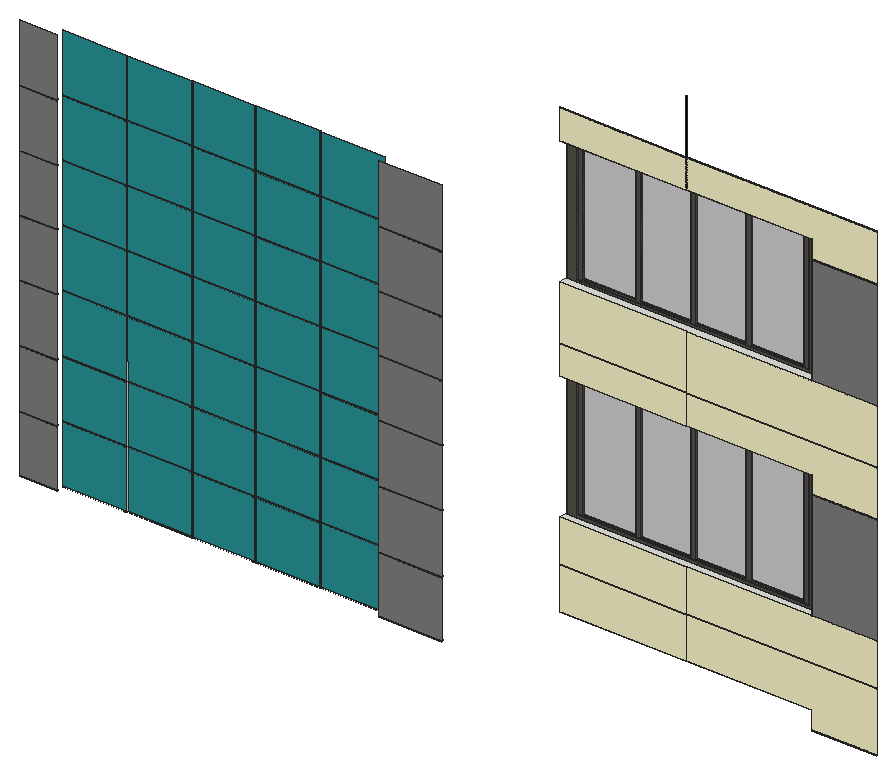
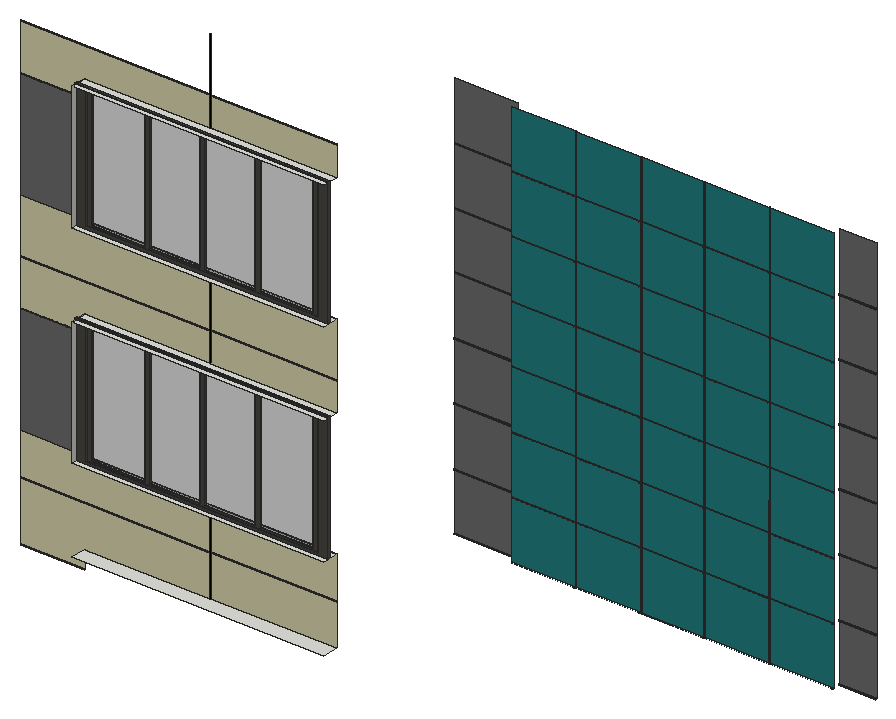
# SketchUp Ruby script. Lengths in inches.
U = 1.inch
M = Sketchup.active_model
def pt(a) = Geom::Point3d.new(a.map { |v| v * U })
def face(e, loops, mat)
  f = e.add_face(loops[0].map { |a| pt(a) })
  loops[1..].each { |l| e.add_face(l.map { |a| pt(a) }).erase! }
  f.material = f.back_material = mat if mat
  f
end
# faces: each face lists its corners as indices into pts; further lists are holes
def faces(e, pts, list, mat = nil) = list.each { |f| face(e, (f[0].is_a?(Array) ? f : [f]).map { |l| l.map { |i| pts[i] } }, mat) }
# xy, xz, yz: faces in a plane at the given z, y or x. An outline is a flat list of corners, or four numbers for a rectangle; further outlines are holes
def ring(l) = l.size == 4 ? [[l[0], l[1]], [l[2], l[1]], [l[2], l[3]], [l[0], l[3]]] : l.each_slice(2).to_a
def flat(e, list, mat, &to3) = list.each { |f| face(e, (f[0].is_a?(Array) ? f : [f]).map { |l| ring(l).map { |u, v| to3.(u, v) } }, mat) }
def xy(e, z, list, mat = nil) = flat(e, list, mat) { |x, y| [x, y, z] }
def xz(e, y, list, mat = nil) = flat(e, list, mat) { |x, z| [x, y, z] }
def yz(e, x, list, mat = nil) = flat(e, list, mat) { |y, z| [x, y, z] }
def lines(e, pts, list) = list.each { |a, b| e.add_line(pt(pts[a]), pt(pts[b])) }
# prism: a flat outline (further loops are holes) pulled along v
def prism(e, loops, v, mat = nil)
  f = face(e, loops, mat); d = Geom::Vector3d.new(v.map { |x| x * U })
  f.pushpull(f.normal.samedirection?(d) ? d.length : -d.length)
end
def box(e, o, s, mat = nil) = prism(e, [[o, [o[0] + s[0], o[1], o[2]], [o[0] + s[0], o[1] + s[1], o[2]], [o[0], o[1] + s[1], o[2]]]], [0, 0, s[2]], mat)
def at(x, y, z, deg = 0) = Geom::Transformation.translation(pt([x, y, z])) * Geom::Transformation.rotation(ORIGIN, Z_AXIS, deg.degrees)
def axes(o, x, y, z) = Geom::Transformation.new([*x, 0, *y, 0, *z, 0, *pt(o).to_a, 1])
def part(name) = M.definitions.add(name)
# library, detail: a bought-in or finely detailed component or shape, given as its bounding box
def library(name, o, s) = part(name).tap { |d| box(d.entities, o, s) }
def detail(e, o, s) = box(e.add_group.entities, o, s)
def put(e, d, t, mat = nil) = e.add_instance(d, t).tap { |i| i.material = mat if mat }
def group(e, t, mat = nil) = e.add_group.tap { |g| g.transformation = t; g.material = mat if mat }.entities
root = M.entities
M.materials.add("Aluminum_Anodized_DarkGray").color = [87, 83, 78]
M.materials.add("Glass_Coated_Black").color = [65, 65, 65]
M.materials["Glass_Coated_Black"].alpha = 0.42
M.materials.add("[0050_LemonChiffon]").color = [255, 250, 205]
M.materials.add("[0081_CadetBlue]").color = [40, 149, 153]
M.materials.add("[0133_Gray]").color = [128, 128, 128]
M.materials.add("[0137_Black]").color = [0, 0, 0]
c1 = part("Group\#2")
xy(c1.entities,0,[[0,0,54,3]],"Aluminum_Anodized_DarkGray")
xy(c1.entities,2,[[2.25,0,51.75,1],[2.25,2,51.75,3]],"Aluminum_Anodized_DarkGray")
xy(c1.entities,3,[[3.375,1,14.625,1.5],[15.75,1,26.4375,1.5],[27.5625,1,38.25,1.5],[39.375,1,50.625,1.5],[3.375,1.5,14.625,2],
  [15.75,1.5,26.4375,2],[27.5625,1.5,38.25,2],[39.375,1.5,50.625,2]],"Aluminum_Anodized_DarkGray")
xy(c1.entities,99,[[3.375,1,14.625,1.5],[15.75,1,26.4375,1.5],[26.4375,1,27.5625,2],[27.5625,1,38.25,1.5],[38.25,1,39.375,2],
  [39.375,1,50.625,1.5],[3.375,1.5,14.625,2],[15.75,1.5,26.4375,2],[27.5625,1.5,38.25,2],[39.375,1.5,50.625,2]],"Aluminum_Anodized_DarkGray")
xy(c1.entities,100,[[2.25,0,51.75,1],[2.25,2,51.75,3]],"Aluminum_Anodized_DarkGray")
xy(c1.entities,102,[[0,0,54,3]],"Aluminum_Anodized_DarkGray")
xz(c1.entities,0,[[[0,0,54,102],[2.25,2,51.75,100]]],"Aluminum_Anodized_DarkGray")
xz(c1.entities,1,[[[2.25,2,51.75,100],[39.375,3,50.625,99],[3.375,3,14.625,99],[27.5625,3,38.25,99],[15.75,3,26.4375,99]]],"Aluminum_Anodized_DarkGray")
xz(c1.entities,1.5,[[3.375,3,14.625,99],[15.75,3,27,99],[27.5625,3,38.8125,99],[39.375,3,50.625,99]],"Glass_Coated_Black")
xz(c1.entities,2,[[[2.25,2,51.75,100],[39.375,3,50.625,99],[3.375,3,14.625,99],[27.5625,3,38.25,99],[15.75,3,26.4375,99]]],"Aluminum_Anodized_DarkGray")
xz(c1.entities,3,[[[0,0,54,102],[2.25,2,51.75,100]]],"Aluminum_Anodized_DarkGray")
yz(c1.entities,0,[[0,0,3,102]],"Aluminum_Anodized_DarkGray")
yz(c1.entities,2.25,[[0,2,1,100],[2,2,3,100]],"Aluminum_Anodized_DarkGray")
yz(c1.entities,3.375,[[1,3,1.5,99],[1.5,3,2,99]],"Aluminum_Anodized_DarkGray")
yz(c1.entities,14.625,[[1,3,1.5,99],[1.5,3,2,99]],"Aluminum_Anodized_DarkGray")
yz(c1.entities,15.75,[[1,3,1.5,99],[1.5,3,2,99]],"Aluminum_Anodized_DarkGray")
yz(c1.entities,26.4375,[[1,3,2,99]],"Aluminum_Anodized_DarkGray")
yz(c1.entities,27.5625,[[1,3,1.5,99],[1.5,3,2,99]],"Aluminum_Anodized_DarkGray")
yz(c1.entities,38.25,[[1,3,2,99]],"Aluminum_Anodized_DarkGray")
yz(c1.entities,39.375,[[1,3,1.5,99],[1.5,3,2,99]],"Aluminum_Anodized_DarkGray")
yz(c1.entities,50.625,[[1,3,1.5,99],[1.5,3,2,99]],"Aluminum_Anodized_DarkGray")
yz(c1.entities,51.75,[[0,2,1,100],[2,2,3,100]],"Aluminum_Anodized_DarkGray")
yz(c1.entities,54,[[0,0,3,102]],"Aluminum_Anodized_DarkGray")
p = [[15.75,2,99],[14.625,2,99]]
lines(c1.entities,p,[[0,1]])
xy(root,276.01,[[355.9375,305.1875,499.37,314.1875]])
xy(root,297.46,[[115.9375,221.1875,136.9375,221.6875],[319.9375,221.1875,355.9375,221.6875],[136.79,225.49,173.04,225.6875],[173.33,225.49,210.01,225.6875],[210.51,225.49,246.05,225.6875],
  [246.55,225.49,283.09,225.6875],[283.59,225.49,319.625,225.6875]])
xy(root,297.96,[[115.9375,221.1875,136.9375,221.6875],[319.9375,221.1875,355.9375,221.6875],[136.79,225.49,173.04,225.6875],[173.33,225.49,210.01,225.6875],[210.51,225.49,246.05,225.6875],
  [246.55,225.49,283.09,225.6875],[283.59,225.49,319.625,225.6875]])
xy(root,324,[[355.9375,305.1875,499.37,314.1875]])
xy(root,330.2,[[115.9375,221.1875,136.9375,221.6875],[319.9375,221.1875,355.9375,221.6875]])
xy(root,330.7,[[115.9375,221.1875,136.9375,221.6875],[319.9375,221.1875,355.9375,221.6875],[136.75,225.49,173.04,225.6875],[173.29,225.49,210.01,225.6875],[210.51,225.49,246.05,225.6875],
  [246.55,225.49,283.09,225.6875],[283.59,225.49,319.625,225.6875]])
xy(root,331.2,[[136.75,225.49,173.04,225.6875],[173.29,225.49,210.01,225.6875],[210.51,225.49,246.05,225.6875],[246.55,225.49,283.09,225.6875],[283.59,225.49,319.625,225.6875]])
xy(root,363.94,[[115.9375,221.1875,136.9375,221.6875],[319.9375,221.1875,355.9375,221.6875],[136.71,225.49,173.04,225.6875],[173.25,225.49,210.01,225.6875],[210.51,225.49,246.05,225.6875],
  [246.55,225.49,283.09,225.6875],[283.59,225.49,319.625,225.6875]])
xy(root,364.44,[[115.9375,221.1875,136.9375,221.6875],[319.9375,221.1875,355.9375,221.6875],[136.71,225.49,173.04,225.6875],[173.25,225.49,210.01,225.6875],[210.51,225.49,246.05,225.6875],
  [246.55,225.49,283.09,225.6875],[283.59,225.49,319.625,225.6875]])
xy(root,396,[[355.9375,305.1875,499.37,314.1875]])
xy(root,397.18,[[115.9375,221.1875,136.9375,221.6875],[319.9375,221.1875,355.9375,221.6875],[136.68,225.49,173.04,225.6875],[173.21,225.49,210.01,225.6875],[210.51,225.49,246.05,225.6875],
  [246.55,225.49,283.09,225.6875],[283.59,225.49,319.625,225.6875]])
xy(root,397.68,[[115.9375,221.1875,136.9375,221.6875],[319.9375,221.1875,355.9375,221.6875],[136.67,225.49,173.04,225.6875],[173.21,225.49,210.01,225.6875],[210.51,225.49,246.05,225.6875],
  [246.55,225.49,283.09,225.6875],[283.59,225.49,319.625,225.6875]])
xy(root,430.42,[[115.9375,221.1875,136.9375,221.6875],[319.9375,221.1875,355.9375,221.3125],[136.64,225.49,173.04,225.6875],[173.18,225.49,210.01,225.6875],[210.51,225.49,246.05,225.6875],
  [246.55,225.49,283.09,225.6875],[283.59,225.49,319.625,225.6875]])
xy(root,430.88,[[115.9375,221.1875,136.9375,221.6875]])
xy(root,430.92,[[319.9375,221.1875,355.9375,221.3125],[136.64,225.49,173.04,225.6875],[173.18,225.49,210.01,225.6875],[210.51,225.49,246.05,225.6875],[246.55,225.49,283.09,225.6875],
  [283.59,225.49,319.625,225.6875]])
xy(root,444,[[355.9375,305.1875,499.37,314.1875]])
xy(root,463.16,[[115.9375,221.1875,136.9375,221.6875],[319.9375,221.1875,355.9375,221.3125]])
xy(root,463.66,[[115.9375,221.1875,136.9375,221.6875],[319.9375,221.1875,355.9375,221.3125],[136.6,225.49,173.04,225.6875],[173.14,225.49,210.01,225.6875],[210.51,225.49,246.05,225.6875],
  [246.55,225.49,283.09,225.6875],[283.59,225.49,319.625,225.6875]])
xy(root,464.16,[[136.6,225.49,173.04,225.6875],[173.14,225.49,210.01,225.6875],[210.51,225.49,246.05,225.6875],[246.55,225.49,283.09,225.6875],[283.59,225.49,319.625,225.6875]])
xy(root,496.4,[[115.9375,221.1875,136.9375,221.6875],[319.9375,221.1875,355.9375,221.25]])
xy(root,496.9,[[115.9375,221.1875,136.9375,221.6875],[319.9375,221.1875,355.9375,221.25],[136.5625,225.49,173.04,225.6875],[173.1,225.49,210.01,225.6875],[210.51,225.49,246.05,225.6875],
  [246.55,225.49,283.09,225.6875],[283.59,225.49,319.625,225.6875]])
xy(root,497.4,[[136.5625,225.49,173.04,225.6875],[173.1,225.49,210.01,225.6875],[210.51,225.49,246.05,225.6875],[246.55,225.49,283.09,225.6875],[283.59,225.49,319.625,225.6875]])
xy(root,516.13,[[355.9375,305.1875,499.37,314.1875]])
xz(root,221.1875,[[115.9375,297.96,136.9375,330.2],[319.9375,297.96,355.9375,330.2],[115.9375,330.7,136.9375,363.94],[319.9375,330.7,355.9375,363.94],[115.9375,364.44,136.9375,397.18],
  [319.9375,364.44,355.9375,397.18],[115.9375,397.68,136.9375,430.42],[319.9375,397.68,355.9375,430.42],[115.9375,430.88,136.9375,463.16],[319.9375,430.92,355.9375,463.16],
  [115.9375,463.66,136.9375,496.4],[319.9375,463.66,355.9375,496.4],[115.9375,496.9,136.9375,530.14],[319.9375,496.9,355.9375,530.14]],"[0133_Gray]")
xz(root,221.25,[[319.9375,496.4,355.9375,496.9]])
xz(root,221.3125,[[319.9375,463.16,355.9375,463.66]])
xz(root,221.3125,[[319.9375,430.42,355.9375,430.92]],"[0137_Black]")
xz(root,221.6875,[[115.9375,297.46,136.9375,297.96],[115.9375,330.2,136.9375,330.7],[115.9375,363.94,136.9375,364.44],[115.9375,397.18,136.9375,397.68],[115.9375,430.42,136.9375,430.88],
  [115.9375,463.16,136.9375,463.66],[115.9375,496.4,136.9375,496.9]])
xz(root,221.6875,[[319.9375,297.46,355.9375,297.96],[319.9375,330.2,355.9375,330.7],[319.9375,363.94,355.9375,364.44],[319.9375,397.18,355.9375,397.68]],"[0137_Black]")
xz(root,225.6875,[[136.79,297.96,173.04,297.96,173.04,330.7,136.75,330.7],[173.33,297.96,210.01,297.96,210.01,330.7,173.29,330.7],[210.51,297.96,246.05,330.7],[246.55,297.96,283.09,330.7],[283.59,297.96,319.625,330.7],
  [136.75,331.2,173.04,331.2,173.04,363.94,136.71,363.94],[173.29,331.2,210.01,331.2,210.01,363.94,173.25,363.94],[210.51,331.2,246.05,363.94],[246.55,331.2,283.09,363.94],[283.59,331.2,319.625,363.94],
  [136.71,364.44,173.04,364.44,173.04,397.18,136.68,397.18],[173.25,364.44,210.01,364.44,210.01,397.18,173.21,397.18],[210.51,364.44,246.05,397.18],[246.55,364.44,283.09,397.18],[283.59,364.44,319.625,397.18],
  [136.67,397.68,173.04,397.68,173.04,430.42,136.64,430.42],[173.21,397.68,210.01,397.68,210.01,430.42,173.18,430.42],[210.51,397.68,246.05,430.42],[246.55,397.68,283.09,430.42],[283.59,397.68,319.625,430.42],
  [136.64,430.92,173.04,430.92,173.04,463.66,136.6,463.66],[173.18,430.92,210.01,430.92,210.01,463.66,173.14,463.66],[210.51,430.92,246.05,463.66],[246.55,430.92,283.09,463.66],[283.59,430.92,319.625,463.66],
  [136.6,464.16,173.04,464.16,173.04,496.9,136.5625,496.9],[173.14,464.16,210.01,464.16,210.01,496.9,173.1,496.9],[210.51,464.16,246.05,496.9],[246.55,464.16,283.09,496.9],[283.59,464.16,319.625,496.9],
  [136.5625,497.4,173.04,497.4,173.04,530.14,136.52,530.14],[173.1,497.4,210.01,497.4,210.01,530.14,173.0625,530.14],[210.51,497.4,246.05,530.14],[246.55,497.4,283.09,530.14],[283.59,497.4,319.625,530.14]],"[0081_CadetBlue]")
xz(root,305.1875,[[499.37,265.64,535.9375,266.14],[499.37,386.03,535.9375,386.53],[499.37,505.66,535.9375,506.16]])
xz(root,305.1875,[[499.37,266.14,535.9375,266.14,535.9375,299.5,428.15,299.5,428.15,276.01,499.37,276.01],[355.9375,276.01,427.65,299.5],[355.9375,300,427.65,324],[428.15,300,535.9375,324],[499.37,386.53,535.9375,386.53,535.9375,412.5,428.15,412.5,428.15,396,499.37,396],
  [355.9375,396,427.65,412.5],[355.9375,413,427.65,444],[428.15,413,535.9375,444],[499.37,506.16,535.9375,506.16,535.9375,532.63,428.15,532.63,428.15,516.13,499.37,516.13],[355.9375,516.13,427.65,532.63]],"[0050_LemonChiffon]")
xz(root,305.1875,[[499.37,324,535.9375,386.03],[499.37,444,535.9375,505.66]],"[0133_Gray]")
xz(root,305.1875,[[427.65,276.01,428.15,276.01,428.15,299.5,535.9375,299.5,535.9375,300,428.15,300,428.15,324,427.65,324,427.65,300,355.9375,300,355.9375,299.5,427.65,299.5],[427.65,396,428.15,396,428.15,412.5,535.9375,412.5,535.9375,413,428.15,413,428.15,444,427.65,444,427.65,413,355.9375,413,355.9375,412.5,427.65,412.5],[427.65,516.13,428.15,516.13,428.15,532.63,535.9375,532.63,535.9375,533.13,428.15,533.13,428.15,564,427.65,564,427.65,533.13,355.9375,533.13,355.9375,532.63,427.65,532.63]],"[0137_Black]")
yz(root,136.5625,[[225.49,496.9,225.6875,497.4]])
yz(root,136.6,[[225.49,463.66,225.6875,464.16]])
yz(root,136.64,[[225.49,430.42,225.6875,430.92]])
yz(root,136.71,[[225.49,363.94,225.6875,364.44]])
yz(root,136.75,[[225.49,330.7,225.6875,331.2]])
yz(root,136.79,[[225.49,297.46,225.6875,297.96]])
yz(root,173.04,[[225.49,297.96,225.6875,330.7],[225.49,331.2,225.6875,363.94],[225.49,364.44,225.6875,397.18],[225.49,397.68,225.6875,430.42],[225.49,430.92,225.6875,463.66],
  [225.49,464.16,225.6875,496.9],[225.49,497.4,225.6875,530.14]])
yz(root,210.01,[[225.49,297.96,225.6875,330.7],[225.49,331.2,225.6875,363.94],[225.49,364.44,225.6875,397.18],[225.49,397.68,225.6875,430.42],[225.49,430.92,225.6875,463.66],
  [225.49,464.16,225.6875,496.9],[225.49,497.4,225.6875,530.14]])
yz(root,210.51,[[225.49,297.96,225.6875,330.7],[225.49,331.2,225.6875,363.94],[225.49,364.44,225.6875,397.18],[225.49,397.68,225.6875,430.42],[225.49,430.92,225.6875,463.66],
  [225.49,464.16,225.6875,496.9],[225.49,497.4,225.6875,530.14]])
yz(root,246.05,[[225.49,297.96,225.6875,330.7],[225.49,331.2,225.6875,363.94],[225.49,364.44,225.6875,397.18],[225.49,397.68,225.6875,430.42],[225.49,430.92,225.6875,463.66],
  [225.49,464.16,225.6875,496.9],[225.49,497.4,225.6875,530.14]])
yz(root,246.55,[[225.49,297.96,225.6875,330.7],[225.49,331.2,225.6875,363.94],[225.49,364.44,225.6875,397.18],[225.49,397.68,225.6875,430.42],[225.49,430.92,225.6875,463.66],
  [225.49,464.16,225.6875,496.9],[225.49,497.4,225.6875,530.14]])
yz(root,283.09,[[225.49,297.96,225.6875,330.7],[225.49,331.2,225.6875,363.94],[225.49,364.44,225.6875,397.18],[225.49,397.68,225.6875,430.42],[225.49,430.92,225.6875,463.66],
  [225.49,464.16,225.6875,496.9],[225.49,497.4,225.6875,530.14]])
yz(root,283.59,[[225.49,297.96,225.6875,330.7],[225.49,331.2,225.6875,363.94],[225.49,364.44,225.6875,397.18],[225.49,397.68,225.6875,430.42],[225.49,430.92,225.6875,463.66],
  [225.49,464.16,225.6875,496.9],[225.49,497.4,225.6875,530.14]])
yz(root,319.625,[[225.49,297.46,225.6875,297.96],[225.49,330.7,225.6875,331.2],[225.49,363.94,225.6875,364.44],[225.49,397.18,225.6875,397.68],[225.49,430.42,225.6875,430.92],
  [225.49,463.66,225.6875,464.16],[225.49,496.9,225.6875,497.4]])
yz(root,499.37,[[305.1875,324,314.1875,396],[305.1875,444,314.1875,516.13]])
p = [[173.33,225.6875,297.96],[173.29,225.6875,330.7],[173.29,225.49,330.7],[173.33,225.49,297.96],[173.29,225.6875,331.2],[173.25,225.6875,363.94],
  [173.25,225.49,363.94],[173.29,225.49,331.2],[173.25,225.6875,364.44],[173.21,225.6875,397.18],[173.21,225.49,397.18],[173.25,225.49,364.44],
  [136.67,225.6875,397.68],[136.68,225.6875,397.18],[136.68,225.49,397.18],[136.67,225.49,397.68],[173.21,225.6875,397.68],[173.18,225.6875,430.42],
  [173.18,225.49,430.42],[173.21,225.49,397.68],[173.18,225.6875,430.92],[173.14,225.6875,463.66],[173.14,225.49,463.66],[173.18,225.49,430.92],
  [173.14,225.6875,464.16],[173.1,225.6875,496.9],[173.1,225.49,496.9],[173.14,225.49,464.16],[173.1,225.6875,497.4],[173.0625,225.6875,530.14],
  [173.0625,225.49,530.14],[173.1,225.49,497.4],[499.9375,311.1875,444],[499.37,305.1875,444]]
faces(root,p,[[0,1,2,3],[4,5,6,7],[8,9,10,11],[12,13,14,15],[16,17,18,19],[20,21,22,23],[24,25,26,27],[28,29,30,31]])
lines(root,p,[[32,33]])
put(root,c1,axes([355.9375,309.6875,324],[2.66667,0,0],[0,0.5,0],[0,0,0.71]))
put(root,c1,axes([355.9375,309.6875,444],[2.66667,0,0],[0,0.5,0],[0,0,0.71]))
